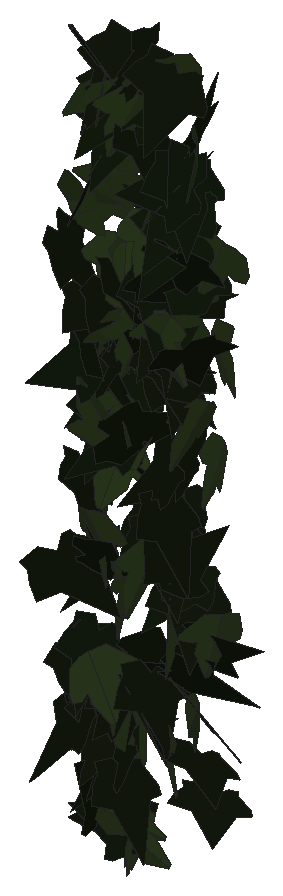
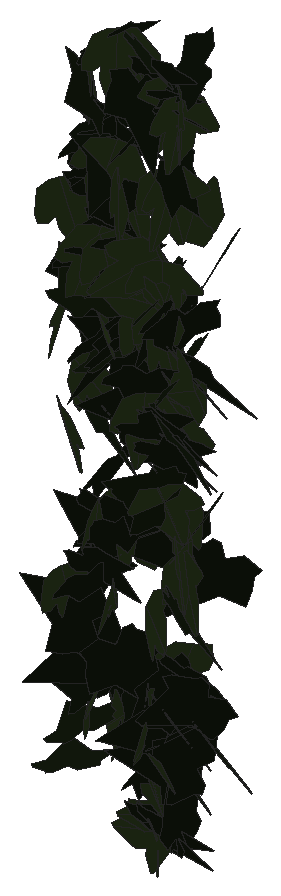
# SketchUp Ruby script. Lengths in inches.
U = 1.inch
M = Sketchup.active_model
def pt(a) = Geom::Point3d.new(a.map { |v| v * U })
def face(e, loops, mat)
  f = e.add_face(loops[0].map { |a| pt(a) })
  loops[1..].each { |l| e.add_face(l.map { |a| pt(a) }).erase! }
  f.material = f.back_material = mat if mat
  f
end
# faces: each face lists its corners as indices into pts; further lists are holes
def faces(e, pts, list, mat = nil) = list.each { |f| face(e, (f[0].is_a?(Array) ? f : [f]).map { |l| l.map { |i| pts[i] } }, mat) }
# xy, xz, yz: faces in a plane at the given z, y or x. An outline is a flat list of corners, or four numbers for a rectangle; further outlines are holes
def ring(l) = l.size == 4 ? [[l[0], l[1]], [l[2], l[1]], [l[2], l[3]], [l[0], l[3]]] : l.each_slice(2).to_a
def flat(e, list, mat, &to3) = list.each { |f| face(e, (f[0].is_a?(Array) ? f : [f]).map { |l| ring(l).map { |u, v| to3.(u, v) } }, mat) }
def xy(e, z, list, mat = nil) = flat(e, list, mat) { |x, y| [x, y, z] }
def xz(e, y, list, mat = nil) = flat(e, list, mat) { |x, z| [x, y, z] }
def yz(e, x, list, mat = nil) = flat(e, list, mat) { |y, z| [x, y, z] }
def lines(e, pts, list) = list.each { |a, b| e.add_line(pt(pts[a]), pt(pts[b])) }
# prism: a flat outline (further loops are holes) pulled along v
def prism(e, loops, v, mat = nil)
  f = face(e, loops, mat); d = Geom::Vector3d.new(v.map { |x| x * U })
  f.pushpull(f.normal.samedirection?(d) ? d.length : -d.length)
end
def box(e, o, s, mat = nil) = prism(e, [[o, [o[0] + s[0], o[1], o[2]], [o[0] + s[0], o[1] + s[1], o[2]], [o[0], o[1] + s[1], o[2]]]], [0, 0, s[2]], mat)
def at(x, y, z, deg = 0) = Geom::Transformation.translation(pt([x, y, z])) * Geom::Transformation.rotation(ORIGIN, Z_AXIS, deg.degrees)
def axes(o, x, y, z) = Geom::Transformation.new([*x, 0, *y, 0, *z, 0, *pt(o).to_a, 1])
def part(name) = M.definitions.add(name)
# library, detail: a bought-in or finely detailed component or shape, given as its bounding box
def library(name, o, s) = part(name).tap { |d| box(d.entities, o, s) }
def detail(e, o, s) = box(e.add_group.entities, o, s)
def put(e, d, t, mat = nil) = e.add_instance(d, t).tap { |i| i.material = mat if mat }
def group(e, t, mat = nil) = e.add_group.tap { |g| g.transformation = t; g.material = mat if mat }.entities
root = M.entities
M.materials.add("efeu1").color = [18, 25, 13]
M.materials.add("efeu2").color = [43, 57, 29]
c1 = part("ivyleaf_9")
p = [[1.54,2.16,1.25],[1.36,2.04,1.19],[-0.21,0.99,0.68],[-0.71,1.11,0.82],[-0.85,0.86,0.67],[-0.8,0.17,0.21],
  [-0.9,-0.01,0.1],[-0.67,-0.16,-0.02],[-0.08,-0.08,-0.05],[-0.03,-0.6,-0.4],[0.65,-0.88,-0.66],[0.83,-0.6,-0.49],
  [1.29,-0.42,-0.43],[1.8125,-0.07,-0.26],[1.21,0.44,0.15]]
faces(c1.entities,p,[[0,1,2,3,4,5,6,7,8,9,10,11,12,13,14]],"efeu1")
c2 = part("ivyleaf_10")
p = [[0,0.5,-0.03],[-0.0625,2.02,-0.43],[-0.19,2.01,-0.46],[-0.54,1.05,-0.29],[-0.52,0.625,-0.18],[-0.83,0.76,-0.28],
  [-1.16,0.64,-0.33],[-1.15,0.33,-0.24],[-0.77,-0.39,0.02],[-0.3,-0.51,0.16],[0.04,-0.48,0.23],[-0.02,2.01,-0.4375],
  [-0.06,2.01,-0.43],[0.04,-0.49,0.23],[0.67,-0.49,0.14],[1.38,0.36,-0.2],[1.375,0.51,-0.24],[0.81,0.65,-0.19],
  [0.62,0.59,-0.15],[0.6,1.09,-0.28],[0.5,1.23,-0.31]]
faces(c2.entities,p,[[0,1,2,3,4,5,6,7,8,9,10],[11,12,0,13,14,15,16,17,18,19,20]],"efeu2")
put(root,c1,axes([584.27,127.14,247.91],[-1.05163,0.23712,-0.34911],[0.32086,-0.15967,-1.07498],[-0.27414,-1.0965,0.08104]))
put(root,c1,axes([583.55,128.3125,256.99],[0.28565,-0.99746,0.28965],[0.05309,-0.28599,-1.03722],[1.03731,0.28932,-0.02667]))
put(root,c1,axes([583.7,126.67,267.49],[0.78296,-0.68215,-0.6481],[-0.43038,0.49013,-1.03582],[0.83674,0.8904,0.07367]))
put(root,c1,axes([584.5,128.46,253.71],[-0.9055,0.50055,-0.20633],[0.16116,-0.13464,-1.0339],[-0.51686,-0.9189,0.0391]))
put(root,c2,axes([584.69,127.8125,254.62],[-0.86208,0.18514,0.74626],[-0.73834,0.1135,-0.88109],[-0.21454,-1.13455,0.03363]))
put(root,c1,axes([583.41,128,249.93],[0.16069,-0.27875,-1.05659],[0.55126,0.94278,-0.16489],[0.9435,-0.50336,0.27629]))
put(root,c2,axes([583.48,128.68,262.93],[0.49288,-0.14872,0.97755],[0.96042,-0.1878,-0.51281],[0.2352,1.07854,0.0455]))
put(root,c1,axes([585.09,127.02,262.76],[-1.00122,0.27768,0.37939],[-0.37051,0.08348,-1.03887],[-0.28943,-1.06744,0.01745]))
put(root,c2,axes([584.53,128.04,255.62],[0.38364,-0.95223,-0.41096],[-0.13943,0.38684,-1.02651],[1.0277,0.40795,0.01414]))
put(root,c1,axes([585.01,128.22,261.04],[-0.80387,0.74194,0.08421],[-0.05683,0.06259,-1.09391],[-0.74454,-0.80585,-0.00743]))
put(root,c1,axes([584.33,128,250.75],[-0.82035,-0.37482,-0.5348],[0.55782,0.04437,-0.88676],[0.33962,-0.97827,0.16468]))
put(root,c1,axes([583.96,126.3,254.65],[-0.15939,-0.3452,-1.08523],[0.3689,1.02107,-0.37897],[1.0774,-0.40068,-0.03079]))
put(root,c1,axes([585.17,128.77,261.2],[-1.08073,0.11662,0.08419],[-0.08588,-0.01134,-1.08681],[-0.11538,-1.08394,0.02043]))
put(root,c1,axes([583.73,128.28,247.05],[0.58633,-0.06134,0.94648],[0.94839,0.05196,-0.58415],[-0.01197,1.11216,0.07949]))
put(root,c1,axes([584.46,128.24,244.11],[0.09564,0.30906,1.32536],[-0.41819,-1.25767,0.32345],[1.29507,-0.42894,0.00656]))
put(root,c2,axes([584.73,127.64,273.57],[-0.45271,-0.98841,-0.31281],[0.20454,0.24947,-1.08429],[1.01635,-0.49047,0.07887]))
put(root,c2,axes([584.79,128.65,258.02],[0.90732,0.52764,-0.28584],[-0.2672,-0.10875,-1.04886],[-0.53732,0.94504,0.0389]))
put(root,c1,axes([584.9,128.68,260.13],[-0.79822,-0.73064,-0.11885],[0.08757,0.08035,-1.08212],[0.73504,-0.80301,-0.00014]))
put(root,c1,axes([584.2,127.19,275.5],[1.01373,-0.51359,0.00329],[0.00148,-0.00435,-1.1364],[0.51359,1.01373,-0.00321]))
put(root,c1,axes([584.6,127.67,265.14],[0.0456,-0.92924,-0.64101],[-0.04075,0.63976,-0.93033],[1.12815,0.06067,-0.00769]))
put(root,c2,axes([585.02,127.42,273.9],[0.63699,-0.90546,-0.33003],[0.007,0.39995,-1.08376],[0.96371,0.59559,0.22602]))
put(root,c1,axes([585.71,127.15,263.07],[-0.9428,0.49306,0.21587],[-0.18241,0.11696,-1.06378],[-0.5064,-0.9601,-0.01872]))
put(root,c1,axes([584.96,128.27,247.6],[-0.46371,-0.93315,0.25954],[-0.0323,-0.27269,-1.03814],[0.96803,-0.45609,0.08969]))
put(root,c2,axes([584.26,126.93,268.9],[-0.40964,-0.26726,1.01753],[1.02504,0.14445,0.4506],[-0.23686,1.08734,0.19024]))
put(root,c1,axes([585.21,127.61,271.2],[-0.61008,0.54223,-0.7783],[0.52484,-0.57786,-0.81399],[-0.79013,-0.80251,0.06025]))
put(root,c1,axes([585.87,127.96,243.8],[-0.7584,0.34454,0.54959],[-0.49285,0.24368,-0.83286],[-0.42174,-0.90435,-0.01503]))
put(root,c1,axes([585.44,129.09,261.01],[-0.83794,-0.67647,0.18147],[-0.15154,-0.10116,-1.07679],[0.68379,-0.85138,-0.01625]))
put(root,c1,axes([585.67,127.66,248.64],[-0.93934,0.38883,-0.1026],[0.09631,-0.03559,-1.01663],[-0.39044,-0.94426,-0.00393]))
put(root,c2,axes([585.74,126.88,259.86],[-1.09902,0.10035,-0.53258],[-0.53236,0.02561,1.1034],[0.1015,1.22099,0.02062]))
put(root,c2,axes([585.28,128.21,266.85],[-1.01908,-0.47277,0.04115],[0.14854,-0.41036,-1.03599],[0.45071,-0.93371,0.43447]))
put(root,c2,axes([585.65,127.43,270.18],[-0.90882,-0.52271,0.3793],[-0.33679,-0.17511,-1.04831],[0.55105,-0.9691,-0.01515]))
put(root,c2,axes([584.9,127.21,255.5],[-0.50795,0.43245,-0.82649],[0.47506,-0.68996,-0.65298],[-0.80275,-0.68195,0.13655]))
put(root,c1,axes([584.69,127.6,262.98],[0.69952,-0.96596,-0.07866],[-0.00115,0.09619,-1.19136],[0.96915,0.69733,0.05536]))
put(root,c2,axes([585.09,128.9,253.09],[0.35399,-0.92361,0.58295],[0.38615,-0.46739,-0.97501],[1.02166,0.49667,0.16653]))
put(root,c2,axes([585.45,127.8125,264.17],[-0.0331,-1.10707,0.13559],[0.00743,-0.13587,-1.10751],[1.11532,-0.03195,0.0114]))
put(root,c1,axes([585.05,127.76,265.43],[0.36733,-0.80974,-0.66246],[-0.2276,0.62344,-0.88825],[1.02114,0.43024,0.04033]))
put(root,c1,axes([585.98,127.74,259.76],[-1.06376,0.14027,0.07765],[-0.08291,-0.03535,-1.07199],[-0.13723,-1.06601,0.04576]))
put(root,c1,axes([586.27,127.7,243.53],[-0.54121,0.34094,0.81684],[-0.76212,0.30741,-0.63327],[-0.45014,-0.93039,0.09008]))
put(root,c2,axes([585.38,127.49,270.1],[-0.25327,-1.02607,-0.4364],[0.26263,0.38003,-1.04595],[1.08365,-0.33192,0.1515]))
put(root,c2,axes([585.39,128.71,246.875],[1.01028,-0.4841,-0.01279],[-0.011,0.00663,-1.12028],[0.48414,1.01034,0.00123]))
put(root,c1,axes([584.92,127.8,248.07],[0.52676,0.29768,0.86087],[0.69855,0.5062,-0.60248],[-0.58458,0.87312,0.05579]))
put(root,c2,axes([586.19,127.54,260.33],[0.6827,-0.09238,-0.97578],[-0.96616,0.1367,-0.68891],[0.16495,1.18302,0.00341]))
put(root,c2,axes([585.88,127.39,248.13],[-0.15631,0.29869,1.16812],[-0.52979,1.04108,-0.3371],[-1.08307,-0.55236,-0.00369]))
put(root,c1,axes([586.08,127.4,247.03],[-1.08854,0.43712,-0.24968],[0.22922,-0.0992,-1.17301],[-0.44818,-1.1124,0.00649]))
put(root,c1,axes([585.83,127.89,275.14],[-1.05753,-0.3638,-0.23365],[0.24725,-0.00234,-1.11543],[0.3547,-1.08304,0.0809]))
put(root,c2,axes([585.47,126.51,256.36],[-1.01245,0.33621,-0.32005],[0.30812,-0.08757,-1.06673],[-0.34716,-1.05821,-0.01341]))
put(root,c2,axes([585.67,127.3,273.87],[-0.6915,-0.87433,-0.18508],[0.19195,0.08325,-1.11045],[0.87284,-0.71099,0.09758]))
put(root,c2,axes([585.375,126.51,250.39],[0.4576,0.96832,0.32768],[0.15035,0.29135,-1.07094],[-1.01114,0.48154,-0.01095]))
put(root,c1,axes([584.875,127.82,249.36],[0.77836,0.52253,-0.49096],[0.41234,0.2666,0.93746],[0.58656,-0.88081,-0.00751]))
put(root,c1,axes([584.86,128.71,257.875],[0.60407,-0.58681,0.68899],[0.64062,-0.30788,-0.82387],[0.63927,0.86303,0.17456]))
put(root,c2,axes([585.87,128.46,261.23],[-0.66598,-0.85574,-0.13899],[0.09734,0.10034,-1.08425],[0.86148,-0.67289,0.01507]))
put(root,c1,axes([586.04,127.83,273.86],[-0.96535,-0.58229,0.03801],[0.09585,-0.23071,-1.09999],[0.5756,-0.93814,0.24691]))
put(root,c1,axes([585.99,127.75,273.05],[-0.9331,-0.62216,-0.23747],[0.27862,0.00657,-1.11198],[0.60486,-0.96283,0.14587]))
put(root,c1,axes([586.41,128.02,274.2],[-0.17566,1.11116,-0.12358],[0.0128,-0.12309,-1.12494],[-1.11794,-0.176,0.00653]))
put(root,c2,axes([586.02,127.51,265.68],[1.22791,0.10841,0.13762],[-0.14181,0.04287,1.23147],[0.10288,-1.23486,0.05484]))
put(root,c1,axes([585.21,126.4375,254.96],[0.81268,-0.1147,0.65704],[0.65958,-0.01558,-0.81855],[0.09904,1.04494,0.05992]))
put(root,c1,axes([585.73,128.44,262.64],[-0.50132,-0.85171,-0.59944],[0.39394,0.46078,-0.98415],[0.96413,-0.63114,0.09042]))
put(root,c2,axes([585.3,127.78,265.25],[0.59404,-0.12679,0.98395],[0.99165,0.04183,-0.59329],[0.02946,1.1486,0.13022]))
put(root,c1,axes([585.55,127.82,265.96],[0.52535,-0.9512,0.16756],[0.15491,-0.10529,-1.0834],[0.95334,0.54128,0.08371]))
put(root,c2,axes([585.82,127.92,243.24],[-0.37736,0.19841,-0.94224],[0.40151,-0.88741,-0.34767],[-0.8752,-0.49267,0.24677]))
put(root,c2,axes([585.58,127.36,244.16],[-0.35417,0.04132,-0.98496],[0.98533,-0.01817,-0.35507],[-0.03109,-1.04654,-0.03273]))
put(root,c1,axes([586.93,127.45,275.52],[-0.99413,0.5811,-0.0485],[-0.01036,-0.11345,-1.14688],[-0.58303,-0.98882,0.10308]))
put(root,c2,axes([586.57,127.74,264.42],[-0.30962,-1.00709,0.34545],[-0.0477,-0.34628,-1.05226],[1.06363,-0.3087,0.05338]))
put(root,c2,axes([586.63,127.3125,273.77],[-0.37841,-0.93309,0.51895],[-0.07913,-0.52456,-1.00087],[1.06476,-0.3706,0.11005]))
put(root,c2,axes([585.86,128.27,267.2],[-0.68593,-0.25736,-0.97247],[0.91636,0.32571,-0.73255],[0.41499,-1.1446,0.0102]))
put(root,c1,axes([586.95,128.54,251.01],[0.15079,0.52098,-0.9616],[-0.22893,-0.93416,-0.54201],[-1.06943,0.27343,-0.01955]))
put(root,c2,axes([585.7,128.41,265.61],[-0.13801,0.04989,-1.19769],[1.16608,-0.27388,-0.14578],[-0.27787,-1.1741,-0.01689]))
put(root,c2,axes([585.93,127.75,243.39],[-0.35785,0.03879,-1.06259],[0.98712,-0.40461,-0.3472],[-0.39522,-1.04568,0.09493]))
put(root,c1,axes([586.32,127.08,246.02],[0.2029,-1.07528,-0.22524],[-0.02964,0.22361,-1.09419],[1.09822,0.2047,0.01209]))
put(root,c1,axes([586.41,127.9,272.39],[0.34664,-1.08228,0.0317],[0.02505,-0.02526,-1.13632],[1.08246,0.34717,0.01614]))
put(root,c1,axes([586.4,126.35,260.36],[0.2806,0.69768,-0.91695],[0.11809,0.92137,0.73718],[1.14613,-0.26574,0.14853]))
put(root,c1,axes([586.87,128.76,256.25],[-0.33911,-0.93685,-0.37561],[0.10819,0.36022,-0.99614],[1.00353,-0.35541,-0.01953]))
put(root,c1,axes([586.52,127.8125,248.7],[0.36527,-0.70686,0.73199],[0.34564,-0.6453,-0.79562],[0.95708,0.50281,0.00796]))
put(root,c1,axes([587.32,129.03,257.125],[-0.9029,-0.38438,-0.40311],[0.39175,0.10755,-0.98002],[0.39594,-0.98294,0.05041]))
put(root,c2,axes([587.29,127.29,255.3125],[-0.05833,-0.99344,0.61447],[0.18043,-0.61551,-0.978],[1.1541,0.04602,0.18395]))
put(root,c2,axes([587.36,127.96,269.8],[0.28122,-1.08965,-0.1569],[0.13294,0.19437,-1.11157],[1.09283,0.25676,0.1756]))
put(root,c1,axes([587.14,127.625,250.13],[0.05475,-1.05035,-0.32712],[-0.04812,0.32492,-1.05136],[1.09906,0.06655,-0.02974]))
put(root,c1,axes([586.52,127.63,262.98],[0.48912,-0.27009,1.00515],[0.96069,-0.31014,-0.55082],[0.40044,1.07395,0.09372]))
put(root,c1,axes([587.1875,128.33,255.84],[-0.21053,-1.03674,-0.42166],[0.14798,0.3995,-1.05615],[1.10938,-0.25004,0.06086]))
put(root,c2,axes([587.75,127.68,275.32],[-0.70046,-0.90194,-0.06794],[0.04585,0.05042,-1.14198],[0.90333,-0.70194,0.00528]))
put(root,c2,axes([587.53,127.03,269],[1.11936,-0.08977,-0.02516],[-0.02311,0.02656,-1.12268],[0.09032,1.11933,0.02462]))
put(root,c1,axes([587.4,127.81,266.45],[-0.08653,-1.11858,-0.01331],[-0.001,0.01343,-1.12192],[1.11866,-0.08651,-0.00204]))
put(root,c2,axes([587.89,128.18,266.97],[-0.40819,-1.01331,0.20273],[-0.02696,-0.20746,-1.09122],[1.03304,-0.40581,0.05163]))
put(root,c1,axes([588.2,128.82,254.44],[-0.99475,-0.32974,-0.01532],[0.01595,0.00056,-1.04797],[0.32971,-0.99487,0.00448]))
put(root,c2,axes([587.51,128.98,256.65],[0.02692,-1.02796,0.39253],[0.59722,-0.31614,-0.86885],[0.92418,0.23423,0.55003]))
put(root,c1,axes([587.46,127.875,263.11],[0.49679,-0.73023,-0.66735],[-0.16235,0.67647,-0.86106],[0.97583,0.4843,0.19649]))
put(root,c2,axes([587.77,127.96,270.89],[-0.94444,-0.54668,-0.30729],[0.36002,-0.01779,-1.07486],[0.51349,-0.99301,0.18842]))
put(root,c1,axes([587.85,128.12,265.32],[-0.47776,-0.95182,0.29186],[-0.0677,-0.29191,-1.06282],[0.99325,-0.47772,0.06794]))
put(root,c1,axes([588.27,127.28,267.29],[0.01392,0.89594,-0.78841],[-0.02041,-0.78817,-0.89602],[-1.19327,0.02393,0.00613]))
put(root,c1,axes([588.5625,127.11,259.52],[-0.97774,0.45095,0.05619],[-0.05166,0.02213,-1.07672],[-0.45149,-0.97911,0.00154]))
put(root,c1,axes([588.83,127.71,268.57],[-0.13365,0.07532,1.12914],[-1.0316,0.45932,-0.15274],[-0.46524,-1.04012,0.01432]))
put(root,c2,axes([587.58,127.81,247.64],[-0.46723,0.53618,-0.86189],[0.50002,-0.70413,-0.7091],[-0.88335,-0.68217,0.05449]))
put(root,c1,axes([587.46,128.27,262.77],[-0.04163,-1.04992,0.41765],[0.54204,-0.38526,-0.91447],[0.99144,0.16654,0.5175]))
put(root,c1,axes([588.41,127.17,270.57],[0.10811,0.98378,0.6336],[-0.02993,0.63842,-0.98615],[-1.16978,0.07459,0.08379]))
put(root,c2,axes([587.9,127.8,252.78],[-0.2976,0.76759,-0.76025],[0.17803,-0.74294,-0.8198],[-1.06559,-0.3385,0.07536]))
put(root,c2,axes([587.82,128.3,264.2],[0.58599,-0.64936,0.67422],[0.45895,-0.49395,-0.87464],[0.81584,0.74428,0.00776]))
put(root,c2,axes([587.8,129.2,248.27],[-0.31954,0.0155,1.03507],[0.75511,-0.73751,0.24415],[0.70812,0.79345,0.20672]))
put(root,c2,axes([588.57,127.0625,265.29],[-0.8291,-0.74342,0.05772],[-0.02319,-0.06056,-1.1132],[0.7453,-0.8289,0.02956]))
put(root,c1,axes([588.13,128.76,253.71],[-0.22554,-1.06641,-0.15585],[0.05584,0.14745,-1.08973],[1.07629,-0.23112,0.02388]))
put(root,c1,axes([587.82,127.33,254.47],[-0.21776,-0.0664,1.09538],[1.09194,0.09809,0.22302],[-0.10927,1.1125,0.04572]))
put(root,c1,axes([588.28,127.57,275.21],[-0.42831,-1.03797,0.23762],[0.00476,-0.25799,-1.11836],[1.06481,-0.41636,0.10058]))
put(root,c2,axes([588.37,128.12,267.05],[-0.61429,-0.93142,-0.56717],[0.31383,0.47243,-1.11575],[1.04438,-0.68981,0.00168]))
put(root,c1,axes([588.27,128.55,267.03],[-0.43349,-0.98611,-0.23385],[0.15781,0.18556,-1.07502],[1.00109,-0.45625,0.0682]))
put(root,c1,axes([588.2,128.24,263.36],[-0.13805,-1.06103,0.24216],[0.02122,-0.24668,-1.06873],[1.0881,-0.1298,0.05157]))
put(root,c2,axes([587.99,126.9,265.03],[-0.74189,0.24976,-0.81706],[0.6823,-0.4781,-0.76567],[-0.51423,-0.99469,0.16286]))
put(root,c1,axes([588.78,127.57,269.3],[-0.85186,-0.73929,0.04152],[-0.0487,-0.00721,-1.12761],[0.73885,-0.85284,-0.02646]))
put(root,c1,axes([587.85,128.06,250.39],[0.99371,0.1716,0.53653],[0.53444,0.05658,-1.00794],[-0.178,1.12788,-0.03107]))
put(root,c1,axes([589.18,127.43,259.86],[-0.87545,0.62673,-0.08734],[0.07141,-0.05029,-1.07666],[-0.62874,-0.87836,-0.00068]))
put(root,c1,axes([589.54,126.74,271.38],[-0.89842,0.32367,0.60945],[-0.58242,0.18092,-0.95467],[-0.3701,-1.07044,0.02293]))
put(root,c1,axes([587.89,128.99,265.06],[0.02826,-1.08108,0.16219],[1.06859,-0.00689,-0.23216],[0.23054,0.16449,1.05624]))
put(root,c1,axes([588.29,127.02,257.76],[0.30871,-1.07262,-0.19886],[-0.0788,0.1842,-1.1159],[1.08805,0.31768,-0.02439]))
put(root,c1,axes([588.89,127.52,270.5],[-0.86502,-0.70667,-0.02188],[0.00402,0.02966,-1.1168],[0.707,-0.86479,-0.02043]))
put(root,c1,axes([589.07,127.46,272.72],[0.28569,0.31735,1.06051],[-0.06754,1.09821,-0.31044],[-1.10491,0.01493,0.29318]))
put(root,c1,axes([589.16,126.57,268.61],[0.71815,0.57725,-0.66021],[-0.62493,-0.26183,-0.90871],[-0.61527,0.93971,0.15236]))
put(root,c1,axes([588.71,127.67,271.42],[-0.13303,-1.1131,-0.11797],[0.03824,0.11421,-1.12076],[1.11868,-0.13627,0.02428]))
put(root,c2,axes([589.11,127.86,261.49],[0.0296,-0.93695,0.58434],[0.03871,-0.58331,-0.93726],[1.10355,0.0456,0.0172]))
put(root,c1,axes([588.3125,128.27,249.23],[0.71227,-0.62619,0.52452],[0.41533,-0.32162,-0.94796],[0.70337,0.82402,0.0286]))
put(root,c1,axes([588.67,128.5,247.04],[-0.0383,-0.98422,0.35705],[0.58158,-0.31709,-0.8117],[0.8706,0.16853,0.55794]))
put(root,c1,axes([588.49,128.36,251.56],[0.77898,0.3908,-0.68763],[0.6138,0.30998,0.87151],[0.4988,-0.99175,0.00144]))
put(root,c2,axes([589.45,128.48,259.65],[0.86194,-0.67832,-0.05307],[-0.04287,0.03133,-1.09684],[0.67905,0.863,-0.00189]))
put(root,c2,axes([589.6,128.33,252.78],[-0.39238,-0.94995,0.21409],[0.02239,-0.23956,-1.02191],[0.97352,-0.37737,0.10979]))
put(root,c2,axes([590.08,127.93,268.46],[-0.95689,-0.23761,0.53048],[-0.49787,-0.19228,-0.9842],[0.29998,-1.07706,0.05867]))
put(root,c2,axes([589.79,126.73,272.89],[0.5065,-0.78962,-0.6812],[-0.20149,0.66893,-0.92521],[1.0232,0.5226,0.15501]))
put(root,c1,axes([589.15,128.7,245.46],[-0.31618,-0.96293,0.18054],[0.61734,-0.34313,-0.74898],[0.76075,-0.12177,0.68282]))
put(root,c1,axes([589.8,126.14,265.12],[0.45855,0.9838,-0.15027],[-0.10217,-0.11805,-1.08459],[-0.98995,0.46788,0.04233]))
put(root,c2,axes([589.6875,128.27,264.375],[-0.56173,0.96396,0.23463],[-0.1129,0.20577,-1.11567],[-0.98566,-0.57293,-0.00592]))
